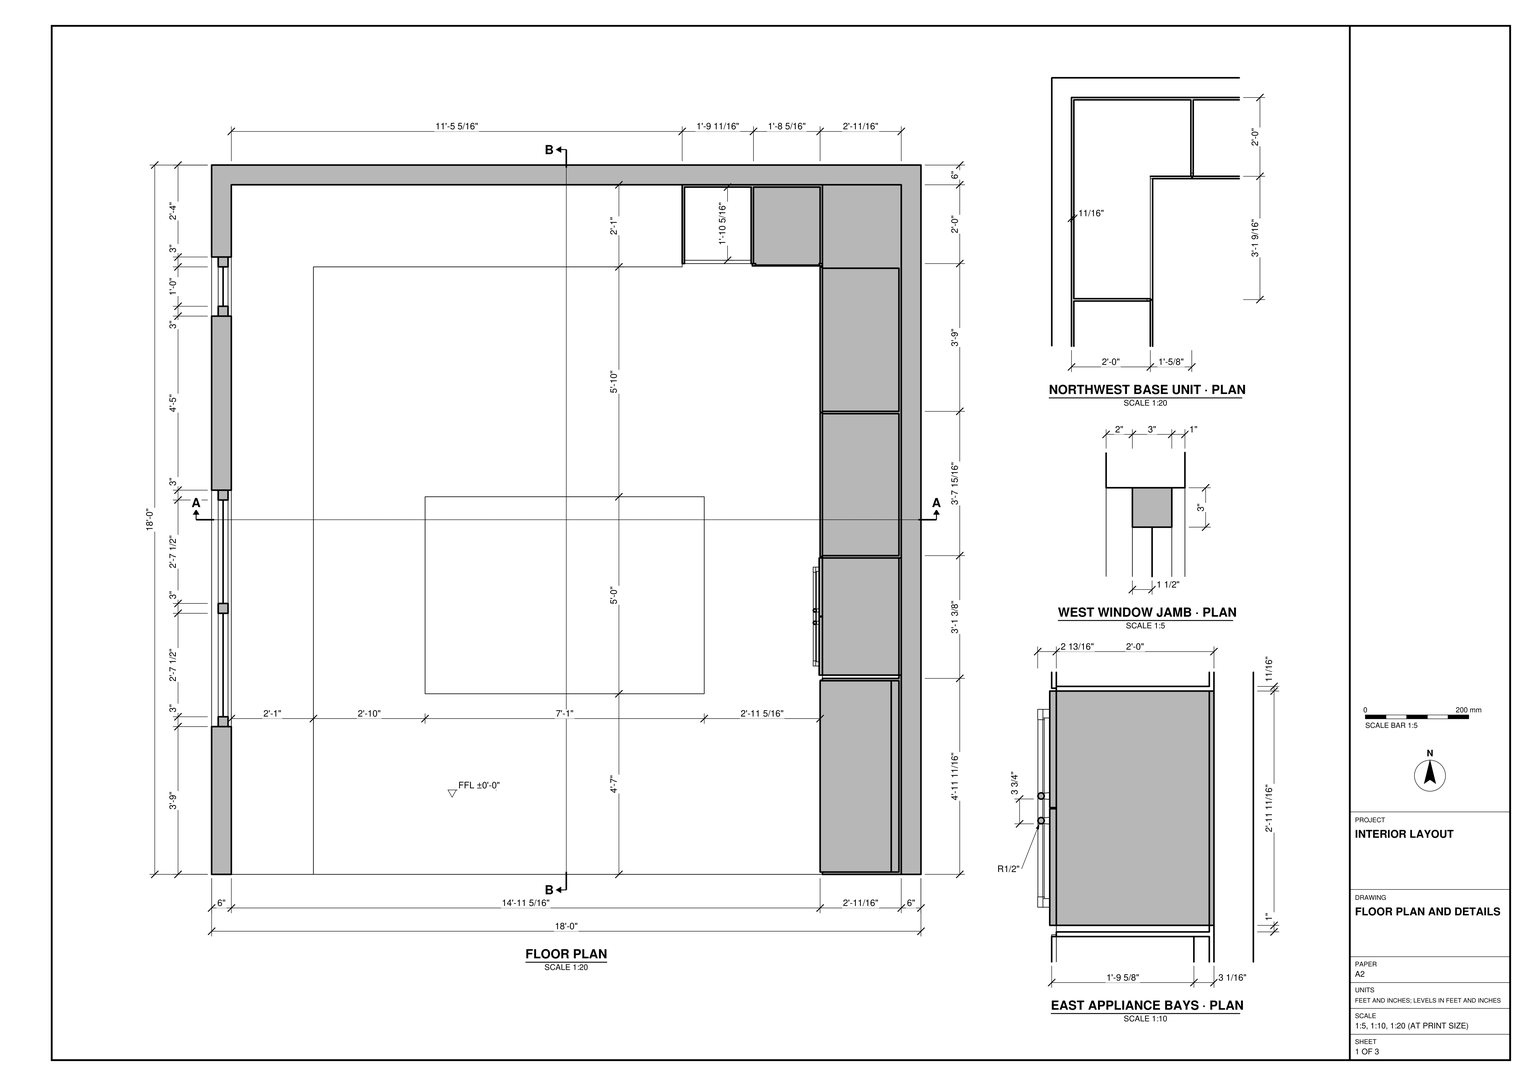
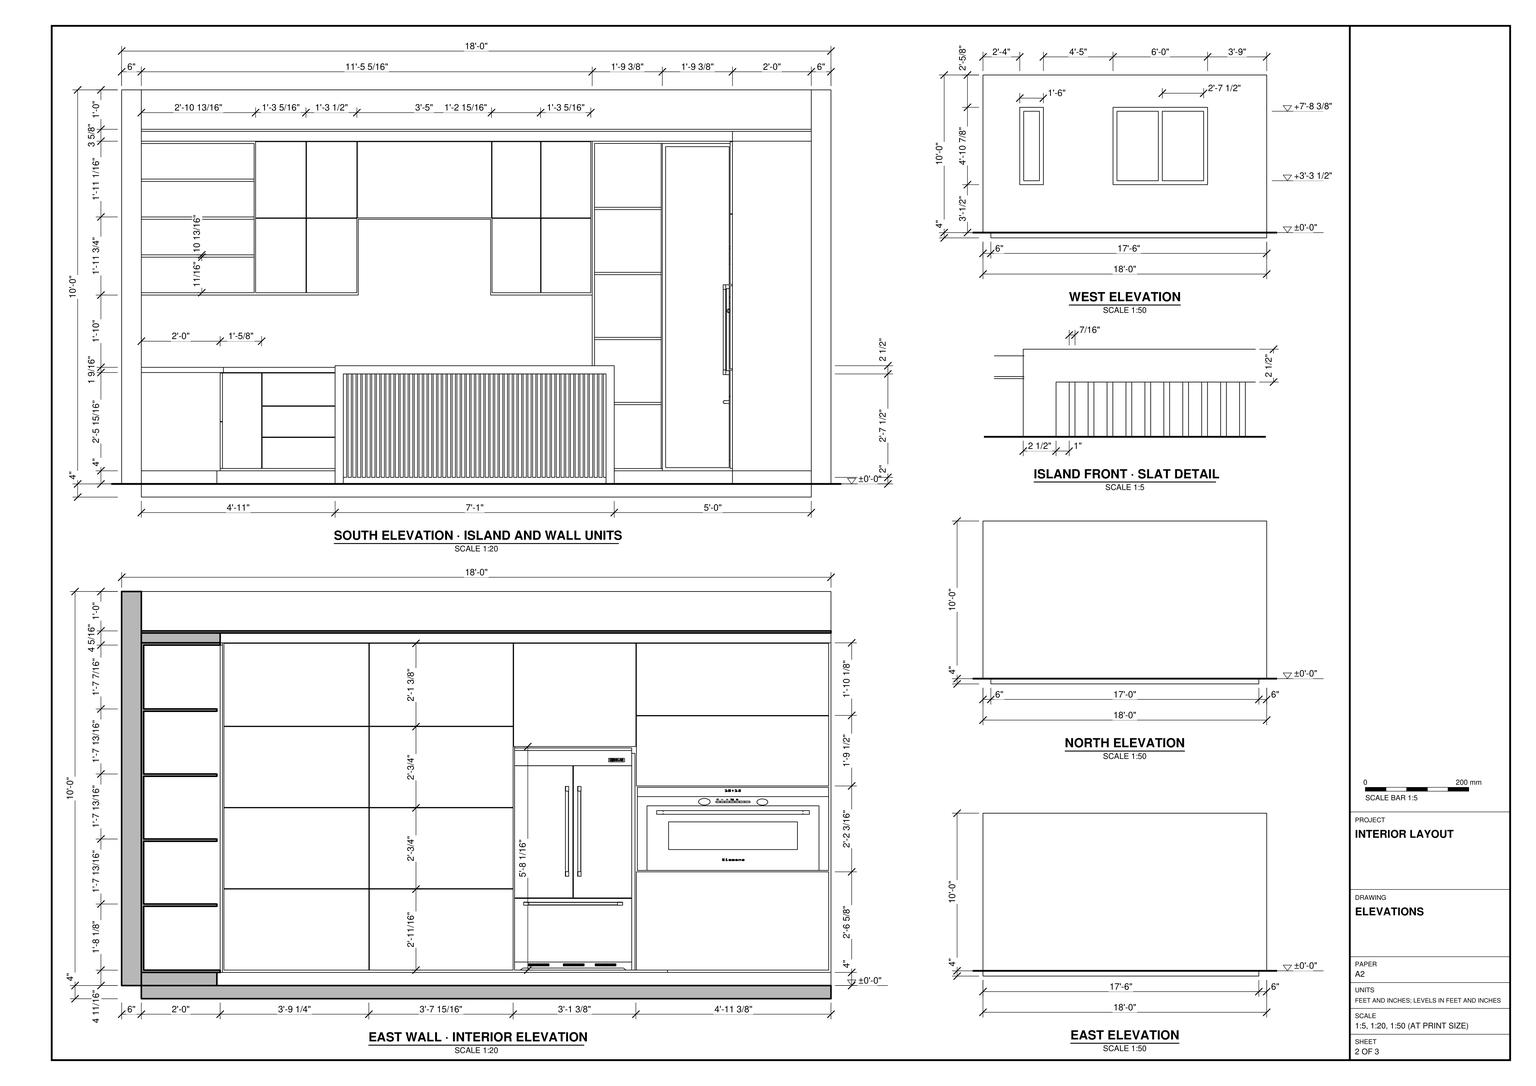
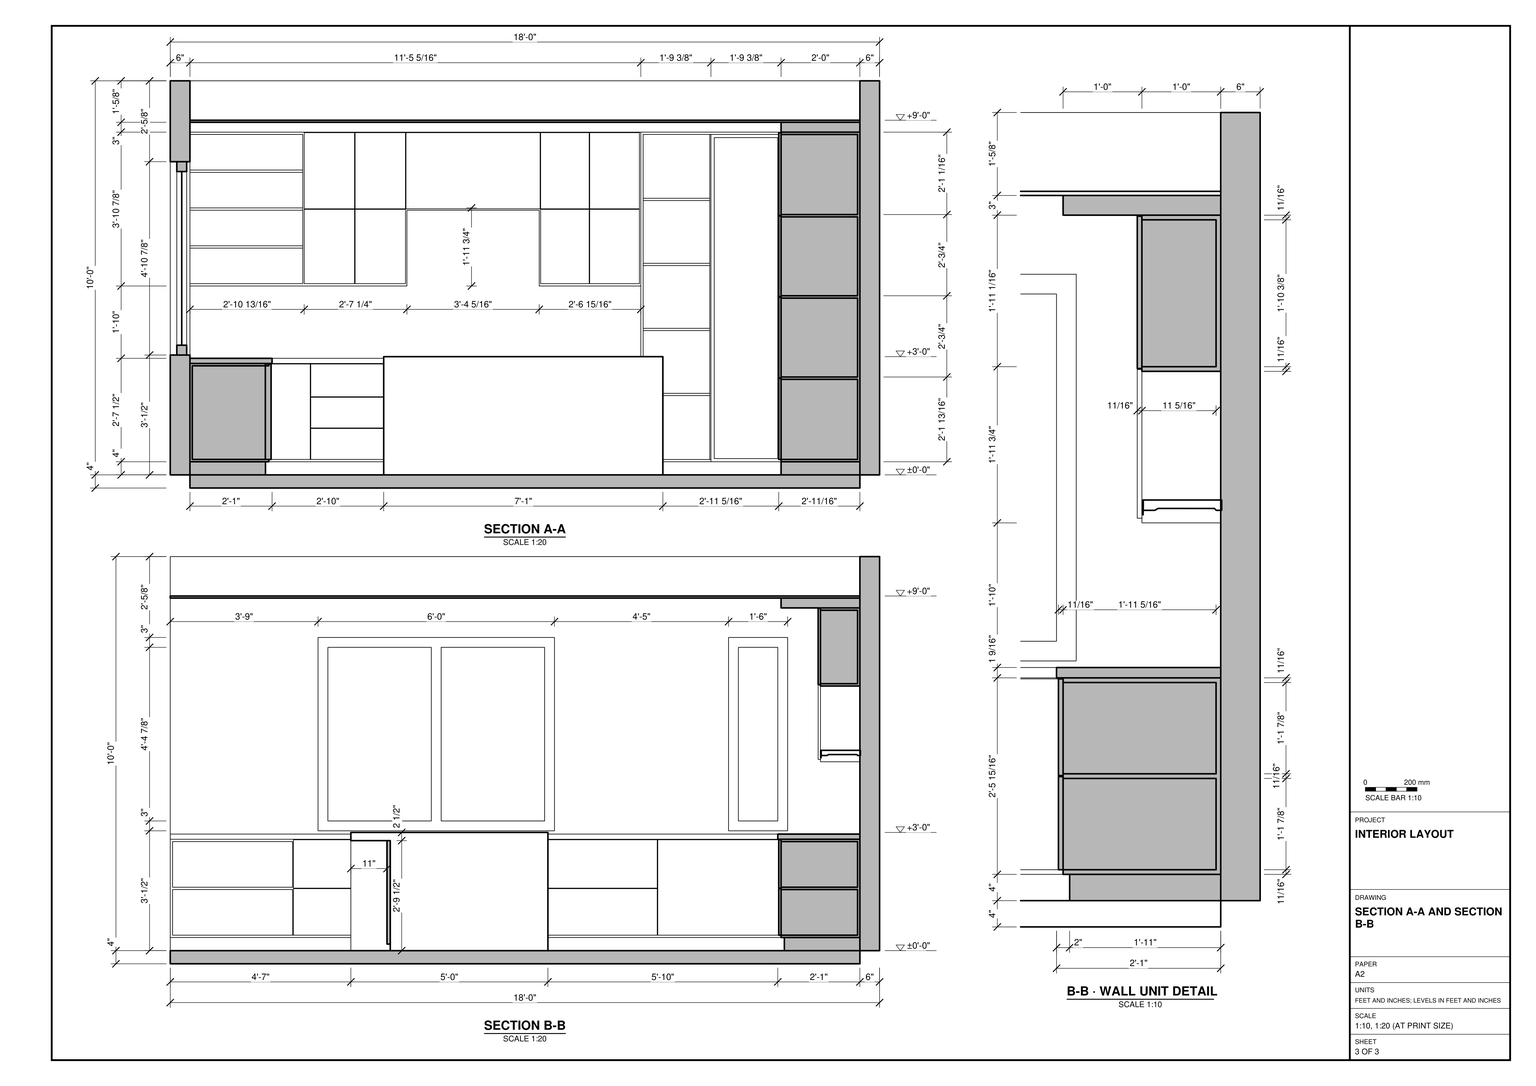
Use task_files/diagram_01.pdf to model the kitchen in SketchUp. Work in feet and inches. The room has an overall footprint of 18'-0" by 18'-0" and an overall height of 10'-4". Set the finished floor at ±0'-0". Model the 4" floor slab and the 6" walls on the north, east and west sides, leaving the south side open as drawn. Follow the sections for the ceiling plane and the west elevation for the narrow window and the wider divided window.

Run the base cabinets and worktop along the west wall and around the north corner. Use the elevations to lay out the drawers, cupboard fronts, open shelves and wall cabinets, including the raised opening in the middle of the north wall units. Build the tall storage and appliance bays along the east wall, with the refrigerator and oven in their indicated positions. Place the 7'-1" by 5'-0" island using the aisle dimensions on the plan. Set its top at +3'-0" and model the framed field of vertical slats on its south face.

Keep shell elements and each furniture or joinery piece in separate groups or components, and use components for repeated parts. Appliances, decor and loose items shown may be any suitable library components. Save one SketchUp model as output_files/kitchen_with_perimeter_cabinetry_and_slatted_island.skp.

# SketchUp Ruby script. Lengths in inches.
U = 1.inch
M = Sketchup.active_model
def pt(a) = Geom::Point3d.new(a.map { |v| v * U })
def face(e, loops, mat)
  f = e.add_face(loops[0].map { |a| pt(a) })
  loops[1..].each { |l| e.add_face(l.map { |a| pt(a) }).erase! }
  f.material = f.back_material = mat if mat
  f
end
# faces: each face lists its corners as indices into pts; further lists are holes
def faces(e, pts, list, mat = nil) = list.each { |f| face(e, (f[0].is_a?(Array) ? f : [f]).map { |l| l.map { |i| pts[i] } }, mat) }
# xy, xz, yz: faces in a plane at the given z, y or x. An outline is a flat list of corners, or four numbers for a rectangle; further outlines are holes
def ring(l) = l.size == 4 ? [[l[0], l[1]], [l[2], l[1]], [l[2], l[3]], [l[0], l[3]]] : l.each_slice(2).to_a
def flat(e, list, mat, &to3) = list.each { |f| face(e, (f[0].is_a?(Array) ? f : [f]).map { |l| ring(l).map { |u, v| to3.(u, v) } }, mat) }
def xy(e, z, list, mat = nil) = flat(e, list, mat) { |x, y| [x, y, z] }
def xz(e, y, list, mat = nil) = flat(e, list, mat) { |x, z| [x, y, z] }
def yz(e, x, list, mat = nil) = flat(e, list, mat) { |y, z| [x, y, z] }
def lines(e, pts, list) = list.each { |a, b| e.add_line(pt(pts[a]), pt(pts[b])) }
# prism: a flat outline (further loops are holes) pulled along v
def prism(e, loops, v, mat = nil)
  f = face(e, loops, mat); d = Geom::Vector3d.new(v.map { |x| x * U })
  f.pushpull(f.normal.samedirection?(d) ? d.length : -d.length)
end
def box(e, o, s, mat = nil) = prism(e, [[o, [o[0] + s[0], o[1], o[2]], [o[0] + s[0], o[1] + s[1], o[2]], [o[0], o[1] + s[1], o[2]]]], [0, 0, s[2]], mat)
def at(x, y, z, deg = 0) = Geom::Transformation.translation(pt([x, y, z])) * Geom::Transformation.rotation(ORIGIN, Z_AXIS, deg.degrees)
def axes(o, x, y, z) = Geom::Transformation.new([*x, 0, *y, 0, *z, 0, *pt(o).to_a, 1])
def part(name) = M.definitions.add(name)
# library, detail: a bought-in or finely detailed component or shape, given as its bounding box
def library(name, o, s) = part(name).tap { |d| box(d.entities, o, s) }
def detail(e, o, s) = box(e.add_group.entities, o, s)
def put(e, d, t, mat = nil) = e.add_instance(d, t).tap { |i| i.material = mat if mat }
def group(e, t, mat = nil) = e.add_group.tap { |g| g.transformation = t; g.material = mat if mat }.entities
root = M.entities
M.materials.add("Aluminum_Polished\#1").color = [83, 85, 85]
M.materials.add("Glass Clear 001").color = [0, 0, 0]
M.materials["Glass Clear 001"].alpha = 0.1
M.materials.add("Glass Milky 001").color = [229, 229, 229]
M.materials["Glass Milky 001"].alpha = 0.37
M.materials.add("[Color_008]1").color = [30, 30, 30]
c1 = library("JFC2290VEM 72_ Cabinet Depth French Door Refrigerator with I",[0,-2.84,0],[35.68,26.84,67.65])
c2 = part("kg")
xy(c2.entities,0,[[[0.24,0,0.21,0.01,0.22,0.04,0.24,0.03,0.29,0.03,0.3,0.04,0.3125,0.04,0.32,0.0625,0.32,0.1,0.3,0.08,0.23,0.08,0.21,0.1,0.2,0.12,0.19,0.13,0.19,0.2,0.2,0.22,0.2,0.24,0.22,0.25,0.24,0.27,0.26,0.27,0.27,0.28,0.3,0.27,0.32,0.26,0.32,0.27,0.35,0.27,0.35,0.05,0.34,0.04,0.33,0.02,0.32,0.01,0.31,0.01,0.29,0],[0.25,0.11,0.3,0.11,0.32,0.13,0.32,0.24,0.3,0.24,0.28,0.25,0.27,0.25,0.26,0.24,0.25,0.24,0.23,0.22,0.23,0.21,0.22,0.18,0.23,0.15,0.24,0.125,0.24,0.12]],[0.02,0.07,0.02,0.35,0.06,0.35,0.06,0.1875,0.13,0.27,0.18,0.27,0.1,0.1875,0.1875,0.07,0.14,0.07,0.07,0.17,0.06,0.16,0.06,0.07]])
c3 = part("12:15")
xy(c3.entities,0,[[0.08,0,0.07,0.01,0.07,0.05,0.18,0.05,0.18,0.38,0.08,0.38,0.08,0.43,0.23,0.43,0.23,0.05,0.29,0.05,0.29,0.1875,0.3,0.19,0.3125,0.2,0.32,0.19,0.33,0.1875,0.34,0.18,0.34,0.02,0.32,0],[0.47,0,0.47,0.21,0.5,0.24,0.69,0.24,0.69,0.38,0.48,0.38,0.48,0.39,0.47,0.39,0.47,0.42,0.48,0.42,0.48,0.43,0.71,0.43,0.73,0.42,0.75,0.38,0.75,0.24,0.74,0.22,0.71,0.19,0.69,0.1875,0.52,0.1875,0.52,0.05,0.74,0.05,0.74,0.04,0.75,0.03,0.74,0.02,0.74,0.01,0.73,0],[1.29,0,1.28,0.01,1.28,0.02,1.27,0.03,1.28,0.04,1.28,0.05,1.39,0.05,1.39,0.38,1.29,0.38,1.29,0.43,1.44,0.43,1.44,0.05,1.5,0.05,1.5,0.1875,1.51,0.19,1.52,0.2,1.53,0.19,1.54,0.1875,1.55,0.18,1.55,0.02,1.53,0],[1.76,0,1.7,0.03,1.69,0.04,1.6875,0.05,1.6875,0.0625,1.69,0.07,1.7,0.08,1.71,0.08,1.73,0.07,1.77,0.06,1.78,0.05,1.91,0.05,1.91,0.1875,1.74,0.1875,1.74,0.43,1.94,0.43,1.95,0.42,1.96,0.42,1.96,0.39,1.95,0.39,1.94,0.38,1.8,0.38,1.8,0.24,1.93,0.24,1.95,0.23,1.96,0.21,1.96,0.03,1.93,0],[0.97,0.07,0.96,0.08,0.97,0.17,1.05,0.17,1.06,0.16,1.0625,0.16,1.07,0.14,1.07,0.1,1.06,0.09,1.06,0.08,1.05,0.07],
  [0.97,0.26,0.96,0.27,0.96,0.35,0.97,0.36,1.05,0.36,1.06,0.35,1.06,0.34,1.07,0.33,1.07,0.29,1.0625,0.28,1.06,0.27,1.05,0.26]])
c4 = part("Siemens")
xy(c4.entities,0,[[0.14,0,0.11,0.01,0.09,0.02,0.07,0.05,0.07,0.09,0.08,0.1,0.11,0.1,0.11,0.09,0.12,0.09,0.12,0.08,0.125,0.07,0.13,0.0625,0.14,0.06,0.14,0.05,0.28,0.05,0.29,0.06,0.29,0.0625,0.28,0.07,0.08,0.33,0.07,0.35,0.07,0.39,0.11,0.43,0.3,0.43,0.34,0.39,0.34,0.34,0.33,0.33,0.31,0.33,0.3,0.34,0.29,0.36,0.27,0.38,0.13,0.38,0.12,0.37,0.125,0.36,0.33,0.1,0.34,0.08,0.34,0.04,0.33,0.02,0.31,0],[0.51,0,0.51,0.01,0.5,0.02,0.5,0.04,0.52,0.06,0.58,0.06,0.58,0.26,0.51,0.26,0.51,0.27,0.5,0.28,0.5,0.3,0.51,0.31,0.51,0.3125,0.53,0.32,0.61,0.32,0.62,0.3125,0.63,0.31,0.63,0.3,0.64,0.29,0.64,0.06,0.69,0.06,0.7,0.05,0.71,0.05,0.72,0.04,0.72,0.02,0.7,0],[[0.98,0,0.92,0.02,0.89,0.05,0.875,0.08,0.87,0.1,0.87,0.22,0.88,0.25,0.89,0.27,0.9,0.28,0.93,0.3,0.95,0.31,0.97,0.3125,1.05,0.3125,1.08,0.31,1.11,0.29,1.14,0.26,1.14,0.25,1.15,0.21,1.15,0.13,1.13,0.12,0.93,0.12,0.93,0.09,0.96,0.06,0.97,0.06,0.98,0.05,1.14,0.05,1.15,0.04,1.15,0.02,1.13,0],[0.93,0.17,1.1,0.17,1.1,0.21,1.06,0.26,0.97,0.26,0.96,0.25,0.94,0.24,0.93,0.23]],[1.29,0,1.27,0.02,1.27,0.3,1.28,0.31,1.29,0.3125,1.3,0.3125,1.31,0.31,1.32,0.29,1.35,0.31,1.375,0.32,1.39,0.3125,1.4,0.31,1.42,0.3,1.43,0.29,1.46,0.31,1.47,0.3125,1.49,0.32,1.51,0.3125,1.53,0.3,1.54,0.28,1.55,0.25,1.56,0.03,1.56,0.02,1.54,0,1.52,0,1.5,0.02,1.5,0.24,1.47,0.25,1.44,0.23,1.44,0.03,1.4375,0.02,1.43,0.01,1.42,0,1.4,0,1.39,0.01,1.39,0.25,1.38,0.26,1.36,0.26,1.32,0.22,1.32,0.01,1.31,0],[[1.78,0,1.75,0.01,1.73,0.02,1.7,0.05,1.6875,0.07,1.68,0.08,1.68,0.22,1.6875,0.25,1.7,0.27,1.73,0.3,1.76,0.31,1.78,0.3125,1.86,0.3125,1.89,0.31,1.95,0.25,1.96,0.21,1.96,0.15,1.95,0.13,1.95,0.125,1.9375,0.12,1.73,0.12,1.73,0.1,1.75,0.08,1.76,0.06,1.78,0.06,1.79,0.05,1.95,0.05,1.95,0.04,1.96,0.03,1.95,0.02,1.95,0.01,1.9375,0],[1.74,0.17,1.9,0.17,1.9,0.23,1.89,0.23,1.875,0.25,1.86,0.26,1.77,0.26,1.74,0.23]],
  [2.1,0,2.08,0.02,2.08,0.3,2.09,0.31,2.1,0.3125,2.11,0.32,2.12,0.3125,2.13,0.31,2.14,0.3,2.14,0.27,2.1875,0.3,2.21,0.3125,2.24,0.32,2.27,0.32,2.3,0.31,2.33,0.29,2.34,0.27,2.35,0.23,2.36,0.03,2.36,0.02,2.34,0,2.32,0,2.3125,0.01,2.31,0.02,2.3,0.03,2.3,0.23,2.29,0.24,2.29,0.25,2.28,0.26,2.23,0.26,2.21,0.25,2.14,0.2,2.14,0.02,2.12,0],[2.54,0,2.51,0.02,2.49,0.03,2.49,0.07,2.5,0.08,2.52,0.08,2.54,0.07,2.55,0.06,2.57,0.05,2.67,0.05,2.68,0.06,2.69,0.0625,2.7,0.07,2.7,0.1,2.52,0.19,2.49,0.22,2.49,0.24,2.5,0.27,2.51,0.29,2.54,0.31,2.5625,0.3125,2.6875,0.3125,2.72,0.31,2.74,0.3,2.76,0.28,2.76,0.25,2.72,0.24,2.7,0.26,2.55,0.26,2.56,0.23,2.7,0.16,2.73,0.15,2.75,0.11,2.76,0.08,2.75,0.07,2.75,0.05,2.74,0.04,2.73,0.02,2.67,0],[0.57,0.38,0.55,0.4,0.55,0.44,0.5625,0.45,0.57,0.46,0.62,0.46,0.63,0.45,0.63,0.44,0.64,0.43,0.64,0.41,0.63,0.4,0.63,0.39,0.62,0.38]])
c5 = part("Built-in compact oven")
xy(c5.entities,0,[[0,-23.39,21.65,0]])
xy(c5.entities,11.97,[[-0.55,-21.02,0,-20.24],[-0.55,-3.15,0,-2.36]])
xy(c5.entities,12.76,[[-0.55,-21.02,0,-20.24],[-0.55,-3.15,0,-2.36]])
xy(c5.entities,14.46,[[-0.12,-13.78,0,-13.125],[-0.12,-13.125,0,-12.47],[-0.12,-12.47,0,-11.91],[-0.12,-11.91,0,-11.29],[-0.12,-11.29,0,-10.68],
  [-0.12,-10.68,0,-10.12],[-0.12,-10.12,0,-9.61]])
xy(c5.entities,14.78,[[-0.12,-13.78,0,-13.125],[-0.12,-13.125,0,-12.47],[-0.12,-12.47,0,-11.91],[-0.12,-11.91,0,-11.29],[-0.12,-11.29,0,-10.68],
  [-0.12,-10.68,0,-10.12],[-0.12,-10.12,0,-9.61]])
xy(c5.entities,15.35,[[-0.24,-8.26,0,-8.08]])
xy(c5.entities,17.72,[[0,-23.39,21.65,0]])
xz(c5.entities,-23.39,[[0,0,21.65,17.72]])
xz(c5.entities,-21.02,[[-0.55,11.97,-0.45,11.98,-0.35,12.02,-0.27,12.08,-0.21,12.17,-0.17,12.26,-0.16,12.36,-0.17,12.46,-0.21,12.56,-0.27,12.64,-0.35,12.7,-0.45,12.74,-0.55,12.76,-0.65,12.74,-0.75,12.7,-0.83,12.64,-0.89,12.56,-0.93,12.46,-0.94,12.36,-0.93,12.26,-0.89,12.17,-0.83,12.08,-0.75,12.02,-0.65,11.98],[-0.55,11.97,0,12.76]])
xz(c5.entities,-20.24,[[-0.55,11.97,0,12.76]])
xz(c5.entities,-13.78,[[-0.12,14.46,0,14.78]])
xz(c5.entities,-9.61,[[-0.12,14.46,0,14.78]])
xz(c5.entities,-7.49,[[-0.24,14.54,0,14.72]])
xz(c5.entities,-3.15,[[-0.55,11.97,0,12.76]])
xz(c5.entities,-2.36,[[-0.55,11.97,-0.65,11.98,-0.75,12.02,-0.83,12.08,-0.89,12.17,-0.93,12.26,-0.94,12.36,-0.93,12.46,-0.89,12.56,-0.83,12.64,-0.75,12.7,-0.65,12.74,-0.55,12.76,-0.45,12.74,-0.35,12.7,-0.27,12.64,-0.21,12.56,-0.17,12.46,-0.16,12.36,-0.17,12.26,-0.21,12.17,-0.27,12.08,-0.35,12.02,-0.45,11.98],[-0.55,11.97,0,12.76]])
xz(c5.entities,0,[[0,0,21.65,17.72]])
yz(c5.entities,-0.55,[[-21.02,11.97,-20.24,12.76],[-3.15,11.97,-2.36,12.76]])
yz(c5.entities,-0.24,[[-15.29,13.92,-15.46,13.95,-15.625,14.01,-15.76,14.125,-15.86,14.26,-15.93,14.43,-15.95,14.6,-15.92,14.77,-15.85,14.93,-15.75,15.07,-15.6,15.17,-15.44,15.24,-15.27,15.26,-15.1,15.23,-14.94,15.16,-14.8,15.05,-14.69,14.91,-14.63,14.75,-14.61,14.58,-14.64,14.4,-14.71,14.24,-14.81,14.11,-14.95,14,-15.12,13.9375],[-8.12,13.94,-8.3,13.95,-8.48,14,-8.64,14.1,-8.77,14.23,-8.85,14.4,-8.9,14.58,-8.89,14.76,-8.84,14.94,-8.74,15.1,-8.61,15.22,-8.44,15.3125,-8.26,15.35,-8.08,15.35,-7.9,15.3,-7.74,15.2,-7.62,15.0625,-7.53,14.9,-7.49,14.72,-7.49,14.54,-7.55,14.36,-7.64,14.2,-7.78,14.07,-7.94,13.99]])
yz(c5.entities,-0.12,[[-13.78,14.46,-13.125,14.78],[-13.125,14.46,-12.47,14.78],[-12.47,14.46,-11.91,14.78],[-11.91,14.46,-11.29,14.78],[-11.29,14.46,-10.68,14.78],
  [-10.68,14.46,-10.12,14.78],[-10.12,14.46,-9.61,14.78]])
yz(c5.entities,0,[[[-22.2,0,-1.18,13.78],[-19.57,4.45,-3.82,10.35],[-21.02,11.97,-20.24,12.76],[-3.15,11.97,-2.36,12.76]],[-19.57,4.45,-3.82,10.35],[-12.23,15.01,-12.26,15.03,-12.28,15.04,-12.3,15.07,-12.3125,15.1,-12.32,15.13,-12.3125,15.16,-12.3,15.1875,-12.28,15.21,-12.26,15.23,-12.2,15.25,-12.14,15.23,-12.12,15.21,-12.1,15.1875,-12.09,15.16,-12.08,15.13,-12.1,15.07,-12.12,15.04,-12.14,15.03,-12.17,15.01],[-9.8125,15.04,-9.84,15.05,-9.87,15.06,-9.9,15.08,-9.91,15.1,-9.93,15.13,-9.93,15.19,-9.91,15.22,-9.9,15.24,-9.87,15.26,-9.84,15.27,-9.8125,15.28,-9.78,15.27,-9.75,15.26,-9.71,15.22,-9.69,15.16,-9.71,15.1,-9.75,15.06,-9.78,15.05]])
yz(c5.entities,0,[[[-23.39,0,-23.39,15.75,0,15.75,0,0,-1.18,0,-1.18,13.78,-22.2,13.78,-22.2,0],[-8.12,13.94,-7.94,13.99,-7.78,14.07,-7.64,14.2,-7.55,14.36,-7.49,14.54,-7.49,14.72,-7.53,14.9,-7.62,15.0625,-7.74,15.2,-7.9,15.3,-8.08,15.35,-8.26,15.35,-8.44,15.3125,-8.61,15.22,-8.74,15.1,-8.84,14.94,-8.89,14.76,-8.9,14.58,-8.85,14.4,-8.77,14.23,-8.64,14.1,-8.48,14,-8.3,13.95],[-15.29,13.92,-15.12,13.9375,-14.95,14,-14.81,14.11,-14.71,14.24,-14.64,14.4,-14.61,14.58,-14.63,14.75,-14.69,14.91,-14.8,15.05,-14.94,15.16,-15.1,15.23,-15.27,15.26,-15.44,15.24,-15.6,15.17,-15.75,15.07,-15.85,14.93,-15.92,14.77,-15.95,14.6,-15.93,14.43,-15.86,14.26,-15.76,14.125,-15.625,14.01,-15.46,13.95],[-13.78,14.46,-9.61,14.78],[-9.8125,15.04,-9.78,15.05,-9.75,15.06,-9.71,15.1,-9.69,15.16,-9.71,15.22,-9.75,15.26,-9.78,15.27,-9.8125,15.28,-9.84,15.27,-9.87,15.26,-9.9,15.24,-9.91,15.22,-9.93,15.19,-9.93,15.13,-9.91,15.1,-9.9,15.08,-9.87,15.06,-9.84,15.05],[-12.23,15.01,-12.17,15.01,-12.14,15.03,-12.12,15.04,-12.1,15.07,-12.08,15.13,-12.09,15.16,-12.1,15.1875,-12.12,15.21,-12.14,15.23,-12.2,15.25,-12.26,15.23,-12.28,15.21,-12.3,15.1875,-12.3125,15.16,-12.32,15.13,-12.3125,15.1,-12.3,15.07,-12.28,15.04,-12.26,15.03]]],"Aluminum_Polished\#1")
yz(c5.entities,0,[[-23.39,15.75,0,17.72]],"[Color_008]1")
yz(c5.entities,21.65,[[-23.39,0,0,17.72]])
# 5 loose lines left out
p = [[-0.75,-21.02,12.02],[-0.83,-21.02,12.08],[-0.83,-2.36,12.08],[-0.75,-2.36,12.02],[-0.55,-21.02,11.97],[-0.65,-21.02,11.98],
  [-0.65,-2.36,11.98],[-0.55,-2.36,11.97],[-0.55,-3.15,11.97],[-0.45,-21.02,11.98],[-0.45,-2.36,11.98],[-0.27,-21.02,12.08],
  [-0.35,-21.02,12.02],[-0.35,-2.36,12.02],[-0.27,-2.36,12.08],[-0.89,-21.02,12.17],[-0.89,-2.36,12.17],[-0.21,-21.02,12.17],
  [-0.21,-2.36,12.17],[-0.93,-21.02,12.26],[-0.93,-2.36,12.26],[-0.17,-21.02,12.26],[-0.17,-2.36,12.26],[-0.94,-21.02,12.36],
  [-0.94,-2.36,12.36],[-0.16,-21.02,12.36],[-0.16,-2.36,12.36],[-0.93,-21.02,12.46],[-0.93,-2.36,12.46],[-0.17,-21.02,12.46],
  [-0.17,-2.36,12.46],[-0.89,-21.02,12.56],[-0.89,-2.36,12.56],[-0.21,-21.02,12.56],[-0.21,-2.36,12.56],[-0.83,-21.02,12.64],
  [-0.83,-2.36,12.64],[-0.75,-21.02,12.7],[-0.75,-2.36,12.7],[-0.35,-21.02,12.7],[-0.27,-21.02,12.64],[-0.27,-2.36,12.64],
  [-0.35,-2.36,12.7],[-0.65,-21.02,12.74],[-0.65,-2.36,12.74],[-0.55,-21.02,12.76],[-0.55,-3.15,12.76],[-0.55,-2.36,12.76],
  [-0.45,-21.02,12.74],[-0.45,-2.36,12.74],[0,-15.46,13.95],[0,-15.625,14.01],[-0.24,-15.625,14.01],[-0.24,-15.46,13.95],
  [0,-15.29,13.92],[-0.24,-15.29,13.92],[0,-15.12,13.9375],[-0.24,-15.12,13.9375],[0,-14.95,14],[-0.24,-14.95,14],
  [0,-8.3,13.95],[0,-8.48,14],[-0.24,-8.48,14],[-0.24,-8.3,13.95],[0,-8.12,13.94],[-0.24,-8.12,13.94],
  [0,-7.94,13.99],[-0.24,-7.94,13.99],[0,-15.76,14.125],[-0.24,-15.76,14.125],[0,-14.81,14.11],[-0.24,-14.81,14.11],
  [0,-8.64,14.1],[-0.24,-8.64,14.1],[0,-7.78,14.07],[-0.24,-7.78,14.07],[0,-15.86,14.26],[-0.24,-15.86,14.26],
  [0,-14.71,14.24],[-0.24,-14.71,14.24],[0,-8.77,14.23],[-0.24,-8.77,14.23],[0,-7.64,14.2],[-0.24,-7.64,14.2],
  [0,-14.64,14.4],[-0.24,-14.64,14.4],[0,-8.85,14.4],[-0.24,-8.85,14.4],[0,-7.55,14.36],[-0.24,-7.55,14.36],
  [0,-15.93,14.43],[-0.24,-15.93,14.43],[0,-15.95,14.6],[-0.24,-15.95,14.6],[0,-14.61,14.58],[-0.24,-14.61,14.58],
  [0,-8.9,14.58],[-0.24,-8.9,14.58],[0,-7.49,14.54],[-0.24,-7.49,14.54],[0,-15.92,14.77],[-0.24,-15.92,14.77],
  [0,-14.63,14.75],[-0.24,-14.63,14.75],[0,-8.89,14.76],[-0.24,-8.89,14.76],[0,-7.53,14.9],[0,-7.49,14.72],
  [-0.24,-7.49,14.72],[-0.24,-7.53,14.9],[0,-15.85,14.93],[-0.24,-15.85,14.93],[0,-14.69,14.91],[-0.24,-14.69,14.91],
  [0,-8.84,14.94],[-0.24,-8.84,14.94],[0,-15.75,15.07],[-0.24,-15.75,15.07],[0,-14.8,15.05],[-0.24,-14.8,15.05],
  [0,-8.74,15.1],[-0.24,-8.74,15.1],[0,-7.62,15.0625],[-0.24,-7.62,15.0625],[0,-15.6,15.17],[-0.24,-15.6,15.17],
  [0,-14.94,15.16],[-0.24,-14.94,15.16],[0,-8.61,15.22],[-0.24,-8.61,15.22],[0,-7.74,15.2],[-0.24,-7.74,15.2],
  [0,-15.44,15.24],[-0.24,-15.44,15.24],[0,-15.27,15.26],[-0.24,-15.27,15.26],[0,-15.1,15.23],[-0.24,-15.1,15.23],
  [0,-8.44,15.3125],[-0.24,-8.44,15.3125],[0,-7.9,15.3],[-0.24,-7.9,15.3],[0,-8.26,15.35],[-0.24,-8.26,15.35],
  [0,-8.08,15.35],[-0.24,-8.08,15.35]]
faces(c5.entities,p,[[0,1,2,3],[4,5,6,7,8],[5,0,3,6],[1,15,16,2],[15,19,20,16],[19,23,24,20],[23,27,28,24],[27,31,32,28],
  [31,35,36,32],[35,37,38,36],[37,43,44,38],[43,45,46,47,44]],"Aluminum_Polished\#1")
faces(c5.entities,p,[[9,4,8,7,10],[11,12,13,14],[12,9,10,13],[17,11,14,18],[21,17,18,22],[25,21,22,26],[29,25,26,30],[33,29,30,34],
  [39,40,41,42],[40,33,34,41],[45,48,49,47,46],[48,39,42,49],[50,51,52,53],[54,50,53,55],[56,54,55,57],[58,56,57,59],
  [60,61,62,63],[64,60,63,65],[66,64,65,67],[51,68,69,52],[70,58,59,71],[61,72,73,62],[74,66,67,75],[68,76,77,69],
  [78,70,71,79],[72,80,81,73],[82,74,75,83],[84,78,79,85],[80,86,87,81],[88,82,83,89],[76,90,91,77],[90,92,93,91],
  [94,84,85,95],[86,96,97,87],[98,88,89,99],[92,100,101,93],[102,94,95,103],[96,104,105,97],[106,107,108,109],[100,110,111,101],
  [112,102,103,113],[104,114,115,105],[110,116,117,111],[118,112,113,119],[114,120,121,115],[122,106,109,123],[116,124,125,117],[126,118,119,127],
  [120,128,129,121],[130,122,123,131],[124,132,133,125],[132,134,135,133],[134,136,137,135],[136,126,127,137],[128,138,139,129],[140,130,131,141],
  [138,142,143,139],[144,140,141,145]])
put(c5.entities,c2,axes([0,-11.41,14.97],[0,-1,0],[0,0,1],[-1,0,0]))
put(c5.entities,c3,axes([0,-10.66,16.8],[0,-1,0],[0,0,1],[-1,0,0]))
put(c5.entities,c4,axes([0,-10.31,2.0625],[0,-1,0],[0,0,1],[-1,0,0]))
c6 = library("Chimney",[0,-0.01,0],[29.73,15.52,29.75])
c7 = part("Group28\#2")
xy(c7.entities,0,[[-6,-26.4375,6,26.4375]])
c8 = part("Group27\#1")
prism(c8.entities,[[[-9,29.4375,0],[9,29.4375,0],[9,-29.4375,0],[-9,-29.4375,0]],[[-6,26.4375,0],[-6,-26.4375,0],[6,-26.4375,0],[6,26.4375,0]]],[0,0,3])
put(c8.entities,c7,at(0,0,1.5),"Glass Clear 001")
c9 = part("Group30\#2")
xy(c9.entities,0,[[-33,-26.4375,-1.5,26.4375],[1.5,-26.4375,33,26.4375]])
c10 = part("Group29\#1")
prism(c10.entities,[[[-36,-29.4375,0],[-36,29.4375,0],[36,29.4375,0],[36,-29.4375,0]],[[-33,-26.4375,0],[-1.5,-26.4375,0],[-1.5,26.4375,0],[-33,26.4375,0]],[[33,-26.4375,0],[33,26.4375,0],[1.5,26.4375,0],[1.5,-26.4375,0]]],[0,0,3])
put(c10.entities,c9,at(0,0,1.5),"Glass Clear 001")
c11 = part("Group\#34")
box(c11.entities,[0,0,0],[1,1,31.5])
p = [[72.0625,198,58.23],[72.0625,198,57.52],[72.0625,210,57.52],[6,117,95.37],[6,45,95.37],[6,45,36.5],
  [6,117,36.5]]
lines(root,p,[[0,1],[1,2],[3,4],[4,5],[5,6],[6,3]])
put(root,c1,at(186,96.35,4.71,-90))
put(root,c5,axes([185.29,58.97,35.0625],[1,0,0],[0,2.49134,0],[0,0,1.42756]))
put(root,c6,axes([72.0625,198,57.52],[1.35527,0,0],[0,0.78365,0],[0,0,0.79931]))
g1 = group(root,at(0,0,0))
xy(g1,0,[[0,0,0,216,216,216,216,0,210,0,210,210,6,210,6,0]])
xy(g1,36.5,[[0,45,6,117],[0,170,6,188]])
xy(g1,95.37,[[0,45,6,117],[0,170,6,188]])
xy(g1,120,[[0,0,6,0,6,210,210,210,210,0,216,0,216,216,0,216]])
xz(g1,0,[[0,0,6,120],[210,0,216,120]])
xz(g1,45,[[0,36.5,6,95.37]])
xz(g1,117,[[0,36.5,6,95.37]])
xz(g1,170,[[0,36.5,6,95.37]])
xz(g1,188,[[0,36.5,6,95.37]])
xz(g1,210,[[6,0,210,120]])
xz(g1,216,[[0,0,216,120]])
yz(g1,0,[[[0,0,216,120],[45,36.5,117,95.37],[170,36.5,188,95.37]]])
yz(g1,6,[[[0,0,210,120],[45,36.5,117,95.37],[170,36.5,188,95.37]]])
yz(g1,210,[[0,0,210,120]])
yz(g1,216,[[0,0,216,120]])
put(g1,c8,axes([2,179,65.93],[0,1,0],[0,0,1],[1,0,0]))
g2 = group(root,at(6,0,0))
box(g2,[0,0,-4],[204,210,4])
g3 = group(root,at(6,0,0))
prism(g3,[[[23,187,0],[23,0,0],[0,0,0],[0,210,0],[204,210,0],[204,0,0],[180,0,0],[180,187,0]]],[0,0,4])
g4 = group(root,at(6,0,4))
xy(g4,0,[[0,0,0,210,137.29,210,137.29,186,24,186,24,0]])
xy(g4,0.71,[[0.71,0.71,24,37.27],[0.71,37.98,24,74.1875],[0.71,74.9,24,111.1],[0.71,111.8125,24,148.02],[0.71,148.73,24,148.73,24,186,36.35,186,36.35,209.29,0.71,209.29],
  [37.0625,186,64.65,209.29],[65.35,186,103.9375,209.29],[104.65,186,136.58,209.29]])
xy(g4,9.86,[[37.0625,186,64.65,209.29],[104.65,186,136.58,209.29]])
xy(g4,10.5625,[[37.0625,186,64.65,209.29],[104.65,186,136.58,209.29]])
xy(g4,14.61,[[0.71,0.71,24,37.27],[0.71,37.98,24,74.1875],[0.71,111.8125,24,148.02],[65.35,186,103.9375,209.29]])
xy(g4,15.31,[[0.71,0.71,24,37.27],[0.71,37.98,24,74.1875],[0.71,111.8125,24,148.02],[65.35,186,103.9375,209.29]])
xy(g4,19.36,[[37.0625,186,64.65,209.29],[104.65,186,136.58,209.29]])
xy(g4,20.07,[[37.0625,186,64.65,209.29],[104.65,186,136.58,209.29]])
xy(g4,29.21,[[0.71,0.71,24,37.27],[0.71,37.98,24,74.1875],[0.71,74.9,24,111.1],[0.71,111.8125,24,148.02],[0.71,148.73,24,209.29],
  [24,186,36.35,209.29],[37.0625,186,64.65,209.29],[65.35,186,103.9375,209.29],[104.65,186,136.58,209.29]])
xy(g4,29.92,[[0,0,24,0,24,186,137.29,186,137.29,210,0,210]])
xz(g4,0,[[0,0,24,29.92]])
xz(g4,0.71,[[0.71,0.71,24,14.61],[0.71,15.31,24,29.21]])
xz(g4,37.27,[[0.71,0.71,24,14.61],[0.71,15.31,24,29.21]])
xz(g4,37.98,[[0.71,0.71,24,14.61],[0.71,15.31,24,29.21]])
xz(g4,74.1875,[[0.71,0.71,24,14.61],[0.71,15.31,24,29.21]])
xz(g4,74.9,[[0.71,0.71,24,29.21]])
xz(g4,111.1,[[0.71,0.71,24,29.21]])
xz(g4,111.8125,[[0.71,0.71,24,14.61],[0.71,15.31,24,29.21]])
xz(g4,148.02,[[0.71,0.71,24,14.61],[0.71,15.31,24,29.21]])
xz(g4,148.73,[[0.71,0.71,24,29.21]])
xz(g4,186,[[[24,0,137.29,0,137.29,29.92,24,29.92,24,29.21,36.35,29.21,36.35,0.71,24,0.71],[37.0625,0.71,37.0625,9.86,64.65,9.86,64.65,0.71,65.35,0.71,65.35,14.61,103.9375,14.61,103.9375,0.71,104.65,0.71,104.65,19.36,136.58,19.36,136.58,20.07,104.65,20.07,104.65,29.21,136.58,29.21,136.58,0.71],[65.35,15.31,103.9375,29.21],[37.0625,20.07,64.65,29.21],[37.0625,10.5625,64.65,19.36]],[104.65,9.86,136.58,10.21],[104.65,10.21,136.58,10.5625]])
xz(g4,209.29,[[0.71,0.71,36.35,29.21],[37.0625,0.71,64.65,9.86],[65.35,0.71,103.9375,14.61],[104.65,0.71,136.58,9.86],[37.0625,10.5625,64.65,19.36],
  [104.65,10.5625,136.58,19.36],[65.35,15.31,103.9375,29.21],[37.0625,20.07,64.65,29.21],[104.65,20.07,136.58,29.21]])
xz(g4,210,[[0,0,137.29,29.92]])
yz(g4,0,[[0,0,210,29.92]])
yz(g4,0.71,[[0.71,0.71,37.27,14.61],[37.98,0.71,74.1875,14.61],[74.9,0.71,111.1,29.21],[111.8125,0.71,148.02,14.61],[148.73,0.71,209.29,29.21],
  [0.71,15.31,37.27,29.21],[37.98,15.31,74.1875,29.21],[111.8125,15.31,148.02,29.21]])
yz(g4,24,[[[0,0,186,0,186,0.71,111.8125,0.71,111.8125,14.61,148.02,14.61,148.02,0.71,148.73,0.71,148.73,29.21,186,29.21,186,29.92,0,29.92],[74.9,0.71,111.1,29.21],[0.71,0.71,0.71,14.61,37.27,14.61,37.27,0.71,37.98,0.71,37.98,14.61,74.1875,14.61,74.1875,0.71],[0.71,15.31,37.27,29.21],[111.8125,15.31,148.02,29.21],[37.98,15.31,74.1875,29.21]]])
yz(g4,36.35,[[186,0.71,209.29,29.21]])
yz(g4,37.0625,[[186,0.71,209.29,9.86],[186,10.5625,209.29,19.36],[186,20.07,209.29,29.21]])
yz(g4,64.65,[[186,0.71,209.29,9.86],[186,10.5625,209.29,19.36],[186,20.07,209.29,29.21]])
yz(g4,65.35,[[186,0.71,209.29,14.61],[186,15.31,209.29,29.21]])
yz(g4,103.9375,[[186,0.71,209.29,14.61],[186,15.31,209.29,29.21]])
yz(g4,104.65,[[186,0.71,209.29,9.86],[186,10.5625,209.29,19.36],[186,20.07,209.29,29.21]])
yz(g4,136.58,[[186,0.71,209.29,9.86],[186,10.5625,209.29,19.36],[186,20.07,209.29,29.21]])
yz(g4,137.29,[[186,0,210,29.92]])
g5 = group(root,at(6,0,33.92))
xy(g5,0,[[0,0,0,210,137.29,210,137.29,185,25,185,25,0]])
xy(g5,1.57,[[0,0,25,0,25,185,137.29,185,137.29,210,0,210]])
xz(g5,0,[[0,0,25,1.57]])
xz(g5,185,[[25,0,137.29,1.57]])
xz(g5,210,[[0,0,137.29,1.57]])
yz(g5,0,[[0,0,210,1.57]])
yz(g5,25,[[0,0,185,1.57]])
yz(g5,137.29,[[185,0,210,1.57]])
g6 = group(root,at(6,0,108))
box(g6,[0,0,-0.63],[204,210,0.63])
g7 = group(root,at(6,198,57.52))
xy(g7,0,[[0,0,66.0625,12],[106.35,0,137.29,12]])
xy(g7,0.71,[[0,0,34.35,11.29],[35.0625,0,49.85,11.29],[50.5625,0,65.35,11.29],[107.0625,0,121.29,11.29],[122,0,136.58,11.29]])
xy(g7,11.54,[[0,1,34.35,11.29]])
xy(g7,12.24,[[0,1,34.35,11.29]])
xy(g7,23.07,[[35.0625,0,49.85,11.29],[50.5625,0,65.35,11.29],[66.0625,0,106.35,12],[107.0625,0,121.29,11.29],[122,0,136.58,11.29],
  [0,1,34.35,11.29]])
xy(g7,23.78,[[35.0625,0,49.85,11.29],[50.5625,0,65.35,11.29],[66.0625,0,106.35,11.29],[107.0625,0,121.29,11.29],[122,0,136.58,11.29],
  [0,1,34.35,11.29]])
xy(g7,34.61,[[0,1,34.35,11.29]])
xy(g7,35.32,[[0,1,34.35,11.29]])
xy(g7,46.14,[[0,0,34.35,11.29],[35.0625,0,49.85,11.29],[50.5625,0,65.35,11.29],[66.0625,0,106.35,11.29],[107.0625,0,121.29,11.29],
  [122,0,136.58,11.29]])
xy(g7,46.85,[[0,0,137.29,12]])
xz(g7,0,[[[0,0,66.0625,0,66.0625,23.07,106.35,23.07,106.35,0,137.29,0,137.29,46.85,0,46.85,0,46.14,34.35,46.14,34.35,0.71,0,0.71],[66.0625,23.78,106.35,46.14],[35.0625,23.78,49.85,46.14],[35.0625,0.71,49.85,23.07],[50.5625,23.78,65.35,46.14],[50.5625,0.71,65.35,23.07],[122,23.78,136.58,46.14],[122,0.71,136.58,23.07],[107.0625,23.78,121.29,46.14],[107.0625,0.71,121.29,23.07]]])
xz(g7,1,[[0,11.54,34.35,12.24],[0,23.07,34.35,23.78],[0,34.61,34.35,35.32]])
xz(g7,11.29,[[0,0.71,34.35,11.54],[35.0625,0.71,49.85,23.07],[50.5625,0.71,65.35,23.07],[107.0625,0.71,121.29,23.07],[122,0.71,136.58,23.07],
  [0,12.24,34.35,23.07],[0,23.78,34.35,34.61],[35.0625,23.78,49.85,46.14],[50.5625,23.78,65.35,46.14],[66.0625,23.78,106.35,46.14],
  [107.0625,23.78,121.29,46.14],[122,23.78,136.58,46.14],[0,35.32,34.35,46.14]])
xz(g7,12,[[0,0,0,46.85,137.29,46.85,137.29,0,106.35,0,106.35,23.07,66.0625,23.07,66.0625,0]])
yz(g7,0,[[0,0,0,0.71,11.29,0.71,11.29,46.14,0,46.14,0,46.85,12,46.85,12,0],[1,11.54,11.29,12.24],[1,23.07,11.29,23.78],[1,34.61,11.29,35.32]])
yz(g7,34.35,[[0,0.71,11.29,11.54],[0,11.54,1,12.24],[0,12.24,11.29,23.07],[0,23.07,1,23.78],[0,23.78,11.29,34.61],
  [0,34.61,1,35.32],[0,35.32,11.29,46.14]])
yz(g7,35.0625,[[0,0.71,11.29,23.07],[0,23.78,11.29,46.14]])
yz(g7,49.85,[[0,0.71,11.29,23.07],[0,23.78,11.29,46.14]])
yz(g7,50.5625,[[0,0.71,11.29,23.07],[0,23.78,11.29,46.14]])
yz(g7,65.35,[[0,0.71,11.29,23.07],[0,23.78,11.29,46.14]])
yz(g7,66.0625,[[0,0,12,23.07],[0,23.78,11.29,46.14]])
yz(g7,106.35,[[0,0,12,23.07],[0,23.78,11.29,46.14]])
yz(g7,107.0625,[[0,0.71,11.29,23.07],[0,23.78,11.29,46.14]])
yz(g7,121.29,[[0,0.71,11.29,23.07],[0,23.78,11.29,46.14]])
yz(g7,122,[[0,0.71,11.29,23.07],[0,23.78,11.29,46.14]])
yz(g7,136.58,[[0,0.71,11.29,23.07],[0,23.78,11.29,46.14]])
yz(g7,137.29,[[0,0,12,46.85]])
g8 = group(root,at(125.29,186,4))
xy(g8,0,[[18,0,60.71,24]])
xy(g8,0.6875,[[18.71,0,39,23.29],[39.71,0,60,23.29]])
xy(g8,20.14,[[18.71,1,39,23.29]])
xy(g8,20.83,[[18.71,1,39,23.29]])
xy(g8,39.94,[[18.71,1,39,23.29]])
xy(g8,40.63,[[18.71,1,39,23.29]])
xy(g8,59.74,[[18.71,1,39,23.29]])
xy(g8,60.43,[[18.71,1,39,23.29]])
xy(g8,79.54,[[18.71,1,39,23.29]])
xy(g8,80.23,[[18.71,1,39,23.29]])
xy(g8,99.68,[[18.71,0,39,23.29],[39.71,0,60,23.29]])
xy(g8,100.37,[[18,0,60.71,24]])
xz(g8,0,[[[18,0,60.71,100.37],[18.71,0.6875,60,99.68]],[39,0.6875,39.71,99.68]])
xz(g8,1,[[18.71,20.14,39,20.83],[18.71,39.94,39,40.63],[18.71,59.74,39,60.43],[18.71,79.54,39,80.23]])
xz(g8,23.29,[[18.71,0.6875,39,20.14],[39.71,0.6875,60,20.37],[39.71,20.6,60,40.17],[18.71,20.83,39,39.94],[39.71,40.4,60,59.97],
  [18.71,40.63,39,59.74],[39.71,60.2,60,79.77],[18.71,60.43,39,79.54],[39.71,80,60,99.68],[18.71,80.23,39,99.68]])
xz(g8,24,[[18,0,60.71,100.37]])
yz(g8,18,[[0,0,24,100.37]])
yz(g8,18.71,[[0,0.6875,23.29,0.6875,23.29,20.14,1,20.14,1,20.83,23.29,20.83,23.29,39.94,1,39.94,1,40.63,23.29,40.63,23.29,59.74,1,59.74,1,60.43,23.29,60.43,23.29,79.54,1,79.54,1,80.23,23.29,80.23,23.29,99.68,0,99.68]])
yz(g8,39,[[0,0.6875,0,99.68,23.29,99.68,23.29,80.23,1,80.23,1,79.54,23.29,79.54,23.29,60.43,1,60.43,1,59.74,23.29,59.74,23.29,40.63,1,40.63,1,39.94,23.29,39.94,23.29,20.83,1,20.83,1,20.14,23.29,20.14,23.29,0.6875]])
yz(g8,39.71,[[0,0.6875,23.29,0.6875,23.29,20.37,1,20.37,1,20.6,23.29,20.6,23.29,40.17,1,40.17,1,40.4,23.29,40.4,23.29,59.97,1,59.97,1,60.2,23.29,60.2,23.29,79.77,1,79.77,1,80,23.29,80,23.29,99.68,0,99.68]])
yz(g8,60,[[0,0.6875,0,99.68,23.29,99.68,23.29,80,1,80,1,79.77,23.29,79.77,23.29,60.2,1,60.2,1,59.97,23.29,59.97,23.29,40.4,1,40.4,1,40.17,23.29,40.17,23.29,20.6,1,20.6,1,20.37,23.29,20.37,23.29,0.6875]])
yz(g8,60.71,[[0,0,24,100.37]])
g9 = group(g8,at(39.71,1,79.77),"Glass Milky 001")
xy(g9,0,[[0,0,20.29,22.29]])
xy(g9,0.23,[[0,0,20.29,22.29]])
xz(g9,0,[[0,0,20.29,0.23]])
g10 = group(g8,at(39.71,1,59.97),"Glass Milky 001")
xy(g10,0,[[0,0,20.29,22.29]])
xy(g10,0.23,[[0,0,20.29,22.29]])
xz(g10,0,[[0,0,20.29,0.23]])
g11 = group(g8,at(39.71,1,40.17),"Glass Milky 001")
xy(g11,0,[[0,0,20.29,22.29]])
xy(g11,0.23,[[0,0,20.29,22.29]])
xz(g11,0,[[0,0,20.29,0.23]])
g12 = group(g8,at(39.71,1,20.37),"Glass Milky 001")
xy(g12,0,[[0,0,20.29,22.29]])
xy(g12,0.23,[[0,0,20.29,22.29]])
xz(g12,0,[[0,0,20.29,0.23]])
g13 = group(root,at(164.65,185.29,4))
prism(g13,[[[21.35,0.71,0],[0,0.71,0],[0,0.71,99.68],[21.35,0.71,99.68]],[[20.35,0.71,0.97],[20.35,0.71,98.71],[1,0.71,98.71],[1,0.71,0.97]]],[0,-0.71,0])
g14 = group(root,at(165.65,185.29,4.97),"Glass Clear 001")
box(g14,[0,0,0],[19.35,0.24,97.74])
g15 = group(root,at(30,37.98,19.31))
box(g15,[0,-0.47,-0.28],[0.71,36.95,14.73])
g16 = group(root,at(30,37.98,4.71))
box(g16,[0,-0.47,0],[0.71,36.95,14.17])
g17 = group(root,at(28.96,74.9,4.71))
box(g17,[0,-0.28,0],[1.75,36.76,29.06])
g18 = group(root,at(30,111.8125,19.31))
box(g18,[0,-0.28,-0.28],[0.71,36.76,14.73])
g19 = group(root,at(30,111.8125,4.71))
box(g19,[0,-0.28,0],[0.71,36.76,14.17])
g20 = group(root,at(30,148.73,4.71))
xy(g20,0,[[0,-0.28,0.71,36.5625],[0,36.5625,12.63,37.27]])
xy(g20,29.06,[[0,-0.28,0.71,-0.28,0.71,36.5625,12.63,36.5625,12.63,37.27,0,37.27]])
xz(g20,-0.28,[[0,0,0.71,29.06]])
xz(g20,36.5625,[[0.71,0,12.63,29.06]])
xz(g20,37.27,[[0,0,12.63,29.06]])
yz(g20,0.71,[[-0.28,0,36.5625,29.06]])
yz(g20,12.63,[[36.5625,0,37.27,29.06]])
g21 = group(root,at(43.0625,185.29,4.71))
box(g21,[-0.28,0,19.08],[28.14,0.71,9.98])
box(g21,[-0.28,0,9.58],[28.14,0.71,9.34])
box(g21,[-0.28,0,0],[28.14,0.71,9.42])
g22 = group(root,at(110.65,185.29,4.71))
box(g22,[-0.28,0,9.58],[32.77,0.71,9.34])
box(g22,[-0.28,0,0],[32.77,0.71,9.42])
xy(g22,19.08,[[-0.28,0,32.49,0.71]])
xy(g22,28.5,[[-0.28,0,0,0.71]])
xy(g22,29.06,[[0,0,32.49,0.71]])
xz(g22,0,[[-0.28,19.08,32.49,19.08,32.49,29.06,0,29.06,0,28.5,-0.28,28.5]])
xz(g22,0.71,[[-0.28,19.08,32.49,28.5],[0,28.5,32.49,29.06]])
yz(g22,-0.28,[[0,19.08,0.71,28.5]])
yz(g22,0,[[0,28.5,0.71,29.06]])
yz(g22,32.49,[[0,19.08,0.71,29.06]])
g23 = group(root,at(71.35,186,19.31))
box(g23,[-0.28,-0.71,-0.28],[39.14,0.71,14.73])
g24 = group(root,at(71.35,185.29,4.71))
box(g24,[-0.28,0,0],[39.14,0.71,14.17])
g25 = group(root,at(6,210,104.37))
prism(g25,[[[0,0,0],[204,0,0],[204,-210,0],[180,-210,0],[180,-24,0],[0,-24,0]]],[0,0,3])
g26 = group(root,at(41.0625,197.29,58.23))
box(g26,[-0.28,0,22.8],[15.35,0.71,23.19])
box(g26,[-0.28,0,0],[15.35,0.71,22.64])
box(g26,[15.22,0,22.8],[15.35,0.71,23.19])
box(g26,[15.22,0,0],[15.35,1.33,22.64])
box(g26,[30.72,0,22.8],[40.85,0.71,23.19])
box(g26,[71.72,0,22.8],[14.78,0.71,23.19])
box(g26,[86.66,0,22.8],[15.14,0.71,23.19])
box(g26,[86.66,0,0],[15.14,0.71,22.64])
box(g26,[71.72,0,0],[14.78,0.71,22.64])
put(root,c10,axes([2,81,65.93],[0,1,0],[0,0,1],[1,0,0]))
g27 = group(root,at(186,0,4))
xy(g27,0,[[0,0,24,210]])
xy(g27,0.71,[[0,0.71,23.29,58.97],[0,59.68,23.29,96.35],[0,97.0625,23.29,140.29],[0,141,23.29,184.58]])
xy(g27,25.09,[[0,97.0625,23.29,140.29],[0,141,23.29,184.58]])
xy(g27,25.8,[[0,97.0625,23.29,140.29],[0,141,23.29,184.58]])
xy(g27,30.35,[[0,0.71,23.29,58.97]])
xy(g27,31.0625,[[0,0.71,23.29,58.97]])
xy(g27,49.83,[[0,97.0625,23.29,140.29],[0,141,23.29,184.58]])
xy(g27,50.54,[[0,97.0625,23.29,140.29],[0,141,23.29,184.58]])
xy(g27,56.35,[[0,0.71,23.29,58.97]])
xy(g27,57.0625,[[0,0.71,23.29,58.97]])
xy(g27,66.71,[[0,59.68,23.29,96.35]])
xy(g27,69.0625,[[0,59.68,23.29,96.35]])
xy(g27,74.57,[[0,97.0625,23.29,140.29],[0,141,23.29,184.58]])
xy(g27,75.28,[[0,97.0625,23.29,140.29],[0,141,23.29,184.58]])
xy(g27,77.83,[[0,0.71,23.29,58.97]])
xy(g27,78.54,[[0,0.71,23.29,58.97]])
xy(g27,99.66,[[0,0.71,23.29,58.97],[0,59.68,23.29,96.35],[0,97.0625,23.29,140.29],[0,141,23.29,184.58]])
xy(g27,100.37,[[0,0,24,210]])
xz(g27,0,[[0,0,24,100.37]])
xz(g27,0.71,[[0,0.71,23.29,30.35],[0,31.0625,23.29,56.35],[0,57.0625,23.29,77.83],[0,78.54,23.29,99.66]])
xz(g27,58.97,[[0,0.71,23.29,30.35],[0,31.0625,23.29,56.35],[0,57.0625,23.29,77.83],[0,78.54,23.29,99.66]])
xz(g27,59.68,[[0,0.71,23.29,66.71],[0,69.0625,23.29,99.66]])
xz(g27,96.35,[[0,0.71,23.29,66.71],[0,69.0625,23.29,99.66]])
xz(g27,97.0625,[[0,0.71,23.29,25.09],[0,25.8,23.29,49.83],[0,50.54,23.29,74.57],[0,75.28,23.29,99.66]])
xz(g27,140.29,[[0,0.71,23.29,25.09],[0,25.8,23.29,49.83],[0,50.54,23.29,74.57],[0,75.28,23.29,99.66]])
xz(g27,141,[[0,0.71,23.29,25.09],[0,25.8,23.29,49.83],[0,50.54,23.29,74.57],[0,75.28,23.29,99.66]])
xz(g27,184.58,[[0,0.71,23.29,25.09],[0,25.8,23.29,49.83],[0,50.54,23.29,74.57],[0,75.28,23.29,99.66]])
xz(g27,210,[[0,0,24,100.37]])
yz(g27,0,[[[0,0,0,100.37,185.29,100.37,185.29,0,49.78,0,49.78,0.71,96.35,0.71,96.35,66.71,59.68,66.71,59.68,0.71,58.97,0.71,58.97,30.35,0.71,30.35,0.71,0.71,49.78,0.71,49.78,0],[97.0625,75.28,140.29,75.28,140.29,99.66,141,99.66,141,75.28,184.58,75.28,184.58,99.66,97.0625,99.66],[97.0625,25.8,140.29,25.8,140.29,49.83,97.0625,49.83,97.0625,50.54,140.29,50.54,140.29,74.57,97.0625,74.57],[0.71,31.0625,58.97,56.35],[0.71,78.54,58.97,99.66],[0.71,57.0625,58.97,77.83],[59.68,69.0625,96.35,99.66],[141,0.71,184.58,25.09],[97.0625,0.71,140.29,25.09],[141,25.8,184.58,49.83],[141,50.54,184.58,74.57]],[185.29,0,210,100.37]])
yz(g27,23.29,[[0.71,0.71,58.97,30.35],[59.68,0.71,96.35,66.71],[97.0625,0.71,140.29,25.09],[141,0.71,184.58,25.09],[97.0625,25.8,140.29,49.83],
  [141,25.8,184.58,49.83],[0.71,31.0625,58.97,56.35],[97.0625,50.54,140.29,74.57],[141,50.54,184.58,74.57],[0.71,57.0625,58.97,77.83],
  [59.68,69.0625,96.35,99.66],[97.0625,75.28,140.29,99.66],[141,75.28,184.58,99.66],[0.71,78.54,58.97,99.66]])
yz(g27,24,[[0,0,210,100.37]])
# 1 loose lines left out
g28 = group(root,at(186,141,79.28))
box(g28,[-0.71,-0.28,-0.28],[0.71,44.14,25.22])
g29 = group(root,at(186,0.71,4.71))
box(g29,[-0.71,140.02,49.56],[0.71,44.13,24.58])
box(g29,[-0.71,140.02,24.82],[0.71,44.13,24.58])
box(g29,[-0.71,140.02,0],[0.71,44.13,24.66])
box(g29,[-0.71,96.08,0],[0.71,43.78,24.66])
box(g29,[-0.71,96.08,24.82],[0.71,43.78,24.58])
box(g29,[-0.71,96.08,49.56],[0.71,43.78,24.58])
box(g29,[-0.71,96.08,74.29],[0.71,43.78,25.21])
box(g29,[-0.71,58.7,68.08],[0.71,37.22,31.42])
box(g29,[-0.71,0,77.56],[0.71,58.54,21.94])
box(g29,[-0.71,0,56.08],[0.71,58.54,21.32])
box(g29,[-0.71,0,0],[0.71,58.54,29.92])
xy(g29,55.65,[[0,0,3.35,47.65]])
# 1 loose lines left out
g30 = group(root,at(65,55,0))
xy(g30,0,[[0,0,0,60,85,60,85,0,82.5,0,82.5,12,2.5,12,2.5,0]])
xy(g30,33.5,[[2.5,0,82.5,12]])
xy(g30,36,[[0,0,85,60]])
xz(g30,0,[[0,0,2.5,0,2.5,33.5,82.5,33.5,82.5,0,85,0,85,36,0,36]])
xz(g30,12,[[2.5,0,82.5,33.5]])
xz(g30,60,[[0,0,85,36]])
yz(g30,0,[[0,0,60,36]])
yz(g30,2.5,[[0,0,12,33.5]])
yz(g30,82.5,[[0,0,12,33.5]])
yz(g30,85,[[0,0,60,36]])
put(root,c11,at(67.5,66,2))
put(root,c11,at(68.94,66,2))
put(root,c11,at(70.38,66,2))
put(root,c11,at(71.82,66,2))
put(root,c11,at(73.26,66,2))
put(root,c11,at(74.7,66,2))
put(root,c11,at(76.15,66,2))
put(root,c11,at(77.59,66,2))
put(root,c11,at(79.03,66,2))
put(root,c11,at(80.47,66,2))
put(root,c11,at(81.91,66,2))
put(root,c11,at(83.35,66,2))
put(root,c11,at(84.79,66,2))
put(root,c11,at(86.23,66,2))
put(root,c11,at(87.67,66,2))
put(root,c11,at(89.11,66,2))
put(root,c11,at(90.55,66,2))
put(root,c11,at(92,66,2))
put(root,c11,at(93.4375,66,2))
put(root,c11,at(94.88,66,2))
put(root,c11,at(96.32,66,2))
put(root,c11,at(97.76,66,2))
put(root,c11,at(99.2,66,2))
put(root,c11,at(100.64,66,2))
put(root,c11,at(102.08,66,2))
put(root,c11,at(103.52,66,2))
put(root,c11,at(104.96,66,2))
put(root,c11,at(106.4,66,2))
put(root,c11,at(107.85,66,2))
put(root,c11,at(109.29,66,2))
put(root,c11,at(110.73,66,2))
put(root,c11,at(112.17,66,2))
put(root,c11,at(113.61,66,2))
put(root,c11,at(115.05,66,2))
put(root,c11,at(116.49,66,2))
put(root,c11,at(117.93,66,2))
put(root,c11,at(119.37,66,2))
put(root,c11,at(120.8125,66,2))
put(root,c11,at(122.25,66,2))
put(root,c11,at(123.7,66,2))
put(root,c11,at(125.14,66,2))
put(root,c11,at(126.58,66,2))
put(root,c11,at(128.02,66,2))
put(root,c11,at(129.46,66,2))
put(root,c11,at(130.9,66,2))
put(root,c11,at(132.34,66,2))
put(root,c11,at(133.78,66,2))
put(root,c11,at(135.22,66,2))
put(root,c11,at(136.66,66,2))
put(root,c11,at(138.1,66,2))
put(root,c11,at(139.55,66,2))
put(root,c11,at(140.99,66,2))
put(root,c11,at(142.43,66,2))
put(root,c11,at(143.87,66,2))
put(root,c11,at(145.31,66,2))
put(root,c11,at(146.75,66,2))
